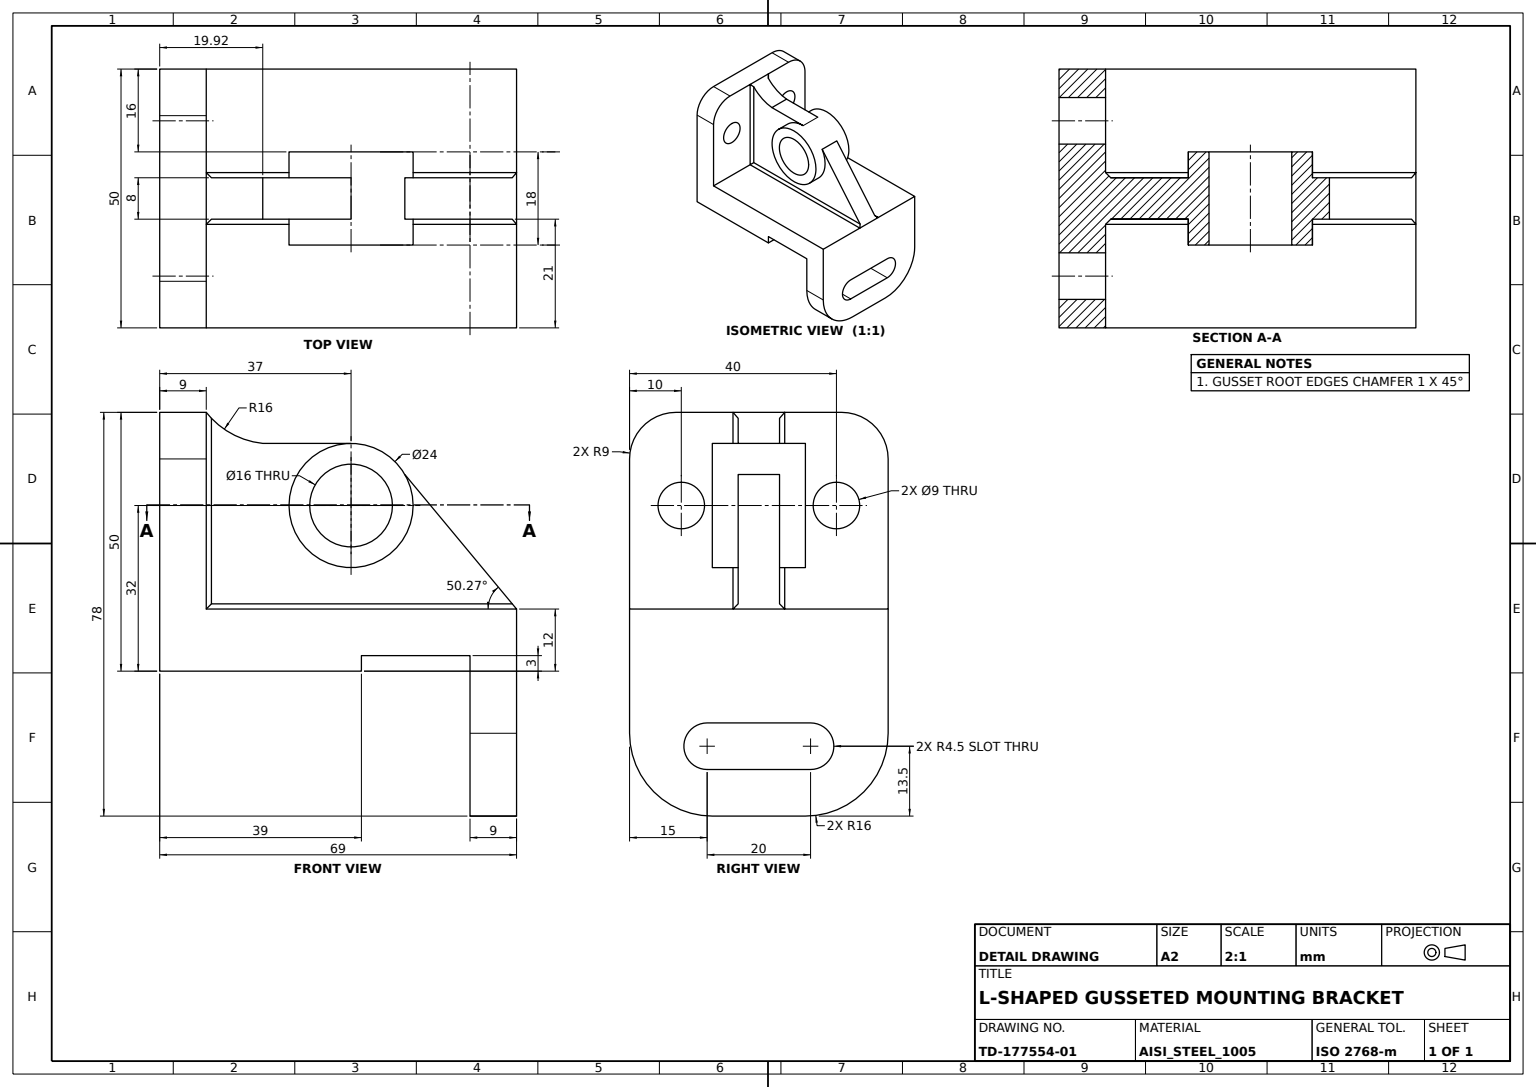
ISO-10303-21;
HEADER;
FILE_DESCRIPTION((''),'2;1');
FILE_NAME('','',(''),(''),'','','');
FILE_SCHEMA(('AUTOMOTIVE_DESIGN'));
ENDSEC;
DATA;
#1=APPLICATION_CONTEXT('');
#2=PRODUCT_CONTEXT('',#1,'mechanical');
#3=PRODUCT('','','',(#2));
#4=PRODUCT_DEFINITION_FORMATION('','',#3);
#5=PRODUCT_DEFINITION_CONTEXT('',#1,'design');
#6=PRODUCT_DEFINITION('','',#4,#5);
#7=PRODUCT_DEFINITION_SHAPE('','',#6);
#8=(LENGTH_UNIT()NAMED_UNIT(*)SI_UNIT(.MILLI.,.METRE.));
#9=(NAMED_UNIT(*)PLANE_ANGLE_UNIT()SI_UNIT($,.RADIAN.));
#10=(NAMED_UNIT(*)SI_UNIT($,.STERADIAN.)SOLID_ANGLE_UNIT());
#11=UNCERTAINTY_MEASURE_WITH_UNIT(LENGTH_MEASURE(0.005),#8,'distance_accuracy_value','');
#12=(GEOMETRIC_REPRESENTATION_CONTEXT(3)GLOBAL_UNCERTAINTY_ASSIGNED_CONTEXT((#11))GLOBAL_UNIT_ASSIGNED_CONTEXT((#8,#9,#10))REPRESENTATION_CONTEXT('',''));
#13=CARTESIAN_POINT('',(9.,-5.,50.));
#14=VERTEX_POINT('',#13);
#15=CARTESIAN_POINT('',(10.,-4.,48.8508));
#16=VERTEX_POINT('',#15);
#17=CARTESIAN_POINT('',(21.556384,7.556384,59.916512));
#18=DIRECTION('',(0.707106781,-0.707106781,0.));
#19=DIRECTION('',(-0.707106781,-0.707106781,0.));
#20=AXIS2_PLACEMENT_3D('',#17,#18,#19);
#21=ELLIPSE('',#20,22.627417,16.);
#22=EDGE_CURVE('',#14,#16,#21,.T.);
#23=ORIENTED_EDGE('',*,*,#22,.F.);
#24=CARTESIAN_POINT('',(9.,-5.,12.));
#25=VERTEX_POINT('',#24);
#26=DIRECTION('',(0.,0.,1.));
#27=VECTOR('',#26,1000.);
#28=LINE('',#13,#27);
#29=EDGE_CURVE('',#25,#14,#28,.T.);
#30=ORIENTED_EDGE('',*,*,#29,.F.);
#31=CARTESIAN_POINT('',(10.,-4.,13.));
#32=VERTEX_POINT('',#31);
#33=CARTESIAN_POINT('',(19.,5.,22.));
#34=DIRECTION('',(0.577350269,0.577350269,0.577350269));
#35=VECTOR('',#34,1000.);
#36=LINE('',#33,#35);
#37=EDGE_CURVE('',#32,#25,#36,.F.);
#38=ORIENTED_EDGE('',*,*,#37,.F.);
#39=CARTESIAN_POINT('',(10.,-4.,12.));
#40=DIRECTION('',(0.,0.,-1.));
#41=VECTOR('',#40,1000.);
#42=LINE('',#39,#41);
#43=EDGE_CURVE('',#16,#32,#42,.T.);
#44=ORIENTED_EDGE('',*,*,#43,.F.);
#45=EDGE_LOOP('',(#23,#30,#38,#44));
#46=FACE_BOUND('',#45,.T.);
#47=CARTESIAN_POINT('',(10.,-4.,32.));
#48=AXIS2_PLACEMENT_3D('',#47,#18,#26);
#49=PLANE('',#48);
#50=ADVANCED_FACE('',(#46),#49,.T.);
#51=CARTESIAN_POINT('',(69.,-9.,-28.));
#52=VERTEX_POINT('',#51);
#53=CARTESIAN_POINT('',(60.,-9.,-28.));
#54=VERTEX_POINT('',#53);
#55=DIRECTION('',(-1.,0.,0.));
#56=VECTOR('',#55,1000.);
#57=LINE('',#51,#56);
#58=EDGE_CURVE('',#52,#54,#57,.T.);
#59=ORIENTED_EDGE('',*,*,#58,.T.);
#60=CARTESIAN_POINT('',(60.,9.,-28.));
#61=VERTEX_POINT('',#60);
#62=DIRECTION('',(0.,1.,0.));
#63=VECTOR('',#62,1000.);
#64=LINE('',#53,#63);
#65=EDGE_CURVE('',#54,#61,#64,.T.);
#66=ORIENTED_EDGE('',*,*,#65,.T.);
#67=CARTESIAN_POINT('',(69.,9.,-28.));
#68=VERTEX_POINT('',#67);
#69=LINE('',#67,#56);
#70=EDGE_CURVE('',#68,#61,#69,.T.);
#71=ORIENTED_EDGE('',*,*,#70,.F.);
#72=LINE('',#51,#63);
#73=EDGE_CURVE('',#52,#68,#72,.T.);
#74=ORIENTED_EDGE('',*,*,#73,.F.);
#75=EDGE_LOOP('',(#59,#66,#71,#74));
#76=FACE_BOUND('',#75,.T.);
#77=DIRECTION('',(1.,0.,0.));
#78=AXIS2_PLACEMENT_3D('',#51,#26,#77);
#79=PLANE('',#78);
#80=ADVANCED_FACE('',(#76),#79,.F.);
#81=CARTESIAN_POINT('',(9.,5.,50.));
#82=VERTEX_POINT('',#81);
#83=CARTESIAN_POINT('',(9.,5.,12.));
#84=VERTEX_POINT('',#83);
#85=LINE('',#83,#41);
#86=EDGE_CURVE('',#82,#84,#85,.T.);
#87=ORIENTED_EDGE('',*,*,#86,.F.);
#88=CARTESIAN_POINT('',(10.,4.,48.8508));
#89=VERTEX_POINT('',#88);
#90=CARTESIAN_POINT('',(21.556384,-7.556384,59.916512));
#91=AXIS2_PLACEMENT_3D('',#90,#19,#18);
#92=ELLIPSE('',#91,22.627417,16.);
#93=EDGE_CURVE('',#89,#82,#92,.F.);
#94=ORIENTED_EDGE('',*,*,#93,.F.);
#95=CARTESIAN_POINT('',(10.,4.,13.));
#96=VERTEX_POINT('',#95);
#97=CARTESIAN_POINT('',(10.,4.,32.));
#98=LINE('',#97,#27);
#99=EDGE_CURVE('',#96,#89,#98,.T.);
#100=ORIENTED_EDGE('',*,*,#99,.F.);
#101=CARTESIAN_POINT('',(26.,-12.,29.));
#102=DIRECTION('',(-0.577350269,0.577350269,-0.577350269));
#103=VECTOR('',#102,1000.);
#104=LINE('',#101,#103);
#105=EDGE_CURVE('',#84,#96,#104,.F.);
#106=ORIENTED_EDGE('',*,*,#105,.F.);
#107=EDGE_LOOP('',(#87,#94,#100,#106));
#108=FACE_BOUND('',#107,.T.);
#109=AXIS2_PLACEMENT_3D('',#83,#19,#40);
#110=PLANE('',#109);
#111=ADVANCED_FACE('',(#108),#110,.F.);
#112=CARTESIAN_POINT('',(69.,10.,-19.));
#113=VERTEX_POINT('',#112);
#114=CARTESIAN_POINT('',(60.,10.,-19.));
#115=VERTEX_POINT('',#114);
#116=LINE('',#112,#56);
#117=EDGE_CURVE('',#113,#115,#116,.T.);
#118=ORIENTED_EDGE('',*,*,#117,.T.);
#119=CARTESIAN_POINT('',(60.,-10.,-19.));
#120=VERTEX_POINT('',#119);
#121=LINE('',#119,#63);
#122=EDGE_CURVE('',#120,#115,#121,.T.);
#123=ORIENTED_EDGE('',*,*,#122,.F.);
#124=CARTESIAN_POINT('',(69.,-10.,-19.));
#125=VERTEX_POINT('',#124);
#126=LINE('',#124,#56);
#127=EDGE_CURVE('',#125,#120,#126,.T.);
#128=ORIENTED_EDGE('',*,*,#127,.F.);
#129=LINE('',#124,#63);
#130=EDGE_CURVE('',#125,#113,#129,.T.);
#131=ORIENTED_EDGE('',*,*,#130,.T.);
#132=EDGE_LOOP('',(#118,#123,#128,#131));
#133=FACE_BOUND('',#132,.T.);
#134=AXIS2_PLACEMENT_3D('',#124,#26,#77);
#135=PLANE('',#134);
#136=ADVANCED_FACE('',(#133),#135,.T.);
#137=CARTESIAN_POINT('',(47.397035,-4.,37.991799));
#138=VERTEX_POINT('',#137);
#139=CARTESIAN_POINT('',(37.,-4.,44.));
#140=VERTEX_POINT('',#139);
#141=CARTESIAN_POINT('',(37.,-4.,32.));
#142=AXIS2_PLACEMENT_3D('',#141,#62,#77);
#143=CIRCLE('',#142,12.);
#144=EDGE_CURVE('',#138,#140,#143,.T.);
#145=ORIENTED_EDGE('',*,*,#144,.T.);
#146=CARTESIAN_POINT('',(19.924011,-4.,44.));
#147=VERTEX_POINT('',#146);
#148=LINE('',#139,#56);
#149=EDGE_CURVE('',#140,#147,#148,.T.);
#150=ORIENTED_EDGE('',*,*,#149,.T.);
#151=CARTESIAN_POINT('',(21.556384,-4.,59.916512));
#152=AXIS2_PLACEMENT_3D('',#151,#62,#77);
#153=CIRCLE('',#152,16.);
#154=EDGE_CURVE('',#147,#16,#153,.T.);
#155=ORIENTED_EDGE('',*,*,#154,.T.);
#156=ORIENTED_EDGE('',*,*,#43,.T.);
#157=CARTESIAN_POINT('',(68.168855,-4.,13.));
#158=VERTEX_POINT('',#157);
#159=CARTESIAN_POINT('',(69.,-4.,13.));
#160=VECTOR('',#77,1000.);
#161=LINE('',#159,#160);
#162=EDGE_CURVE('',#32,#158,#161,.T.);
#163=ORIENTED_EDGE('',*,*,#162,.T.);
#164=CARTESIAN_POINT('',(69.,-4.,12.));
#165=DIRECTION('',(-0.639190848,0.,0.769048152));
#166=VECTOR('',#165,1000.);
#167=LINE('',#164,#166);
#168=EDGE_CURVE('',#158,#138,#167,.T.);
#169=ORIENTED_EDGE('',*,*,#168,.T.);
#170=EDGE_LOOP('',(#145,#150,#155,#156,#163,#169));
#171=FACE_BOUND('',#170,.T.);
#172=AXIS2_PLACEMENT_3D('',#141,#62,#26);
#173=PLANE('',#172);
#174=ADVANCED_FACE('',(#171),#173,.F.);
#175=CARTESIAN_POINT('',(69.,5.,12.));
#176=VERTEX_POINT('',#175);
#177=CARTESIAN_POINT('',(69.,-5.,12.));
#178=VERTEX_POINT('',#177);
#179=CARTESIAN_POINT('',(69.,4.,12.));
#180=DIRECTION('',(0.,-1.,0.));
#181=VECTOR('',#180,1000.);
#182=LINE('',#179,#181);
#183=EDGE_CURVE('',#176,#178,#182,.T.);
#184=ORIENTED_EDGE('',*,*,#183,.T.);
#185=CARTESIAN_POINT('',(69.,-25.,12.));
#186=VERTEX_POINT('',#185);
#187=CARTESIAN_POINT('',(69.,25.,12.));
#188=LINE('',#187,#181);
#189=EDGE_CURVE('',#178,#186,#188,.T.);
#190=ORIENTED_EDGE('',*,*,#189,.T.);
#191=CARTESIAN_POINT('',(69.,-25.,-12.));
#192=VERTEX_POINT('',#191);
#193=LINE('',#185,#41);
#194=EDGE_CURVE('',#186,#192,#193,.T.);
#195=ORIENTED_EDGE('',*,*,#194,.T.);
#196=CARTESIAN_POINT('',(69.,-9.,-12.));
#197=AXIS2_PLACEMENT_3D('',#196,#77,#62);
#198=CIRCLE('',#197,16.);
#199=EDGE_CURVE('',#192,#52,#198,.T.);
#200=ORIENTED_EDGE('',*,*,#199,.T.);
#201=ORIENTED_EDGE('',*,*,#73,.T.);
#202=CARTESIAN_POINT('',(69.,25.,-12.));
#203=VERTEX_POINT('',#202);
#204=CARTESIAN_POINT('',(69.,9.,-12.));
#205=AXIS2_PLACEMENT_3D('',#204,#77,#62);
#206=CIRCLE('',#205,16.);
#207=EDGE_CURVE('',#68,#203,#206,.T.);
#208=ORIENTED_EDGE('',*,*,#207,.T.);
#209=VERTEX_POINT('',#187);
#210=LINE('',#202,#27);
#211=EDGE_CURVE('',#203,#209,#210,.T.);
#212=ORIENTED_EDGE('',*,*,#211,.T.);
#213=EDGE_CURVE('',#209,#176,#188,.T.);
#214=ORIENTED_EDGE('',*,*,#213,.T.);
#215=EDGE_LOOP('',(#184,#190,#195,#200,#201,#208,#212,#214));
#216=FACE_BOUND('',#215,.T.);
#217=CARTESIAN_POINT('',(69.,10.,-10.));
#218=VERTEX_POINT('',#217);
#219=CARTESIAN_POINT('',(69.,10.,-14.5));
#220=AXIS2_PLACEMENT_3D('',#219,#77,#62);
#221=CIRCLE('',#220,4.5);
#222=EDGE_CURVE('',#113,#218,#221,.T.);
#223=ORIENTED_EDGE('',*,*,#222,.F.);
#224=ORIENTED_EDGE('',*,*,#130,.F.);
#225=CARTESIAN_POINT('',(69.,-10.,-10.));
#226=VERTEX_POINT('',#225);
#227=CARTESIAN_POINT('',(69.,-10.,-14.5));
#228=AXIS2_PLACEMENT_3D('',#227,#77,#62);
#229=CIRCLE('',#228,4.5);
#230=EDGE_CURVE('',#226,#125,#229,.T.);
#231=ORIENTED_EDGE('',*,*,#230,.F.);
#232=LINE('',#217,#181);
#233=EDGE_CURVE('',#218,#226,#232,.T.);
#234=ORIENTED_EDGE('',*,*,#233,.F.);
#235=EDGE_LOOP('',(#223,#224,#231,#234));
#236=FACE_BOUND('',#235,.T.);
#237=AXIS2_PLACEMENT_3D('',#196,#77,#40);
#238=PLANE('',#237);
#239=ADVANCED_FACE('',(#216,#236),#238,.T.);
#240=CARTESIAN_POINT('',(60.,-25.,-12.));
#241=VERTEX_POINT('',#240);
#242=CARTESIAN_POINT('',(60.,-9.,-12.));
#243=AXIS2_PLACEMENT_3D('',#242,#77,#62);
#244=CIRCLE('',#243,16.);
#245=EDGE_CURVE('',#241,#54,#244,.T.);
#246=ORIENTED_EDGE('',*,*,#245,.T.);
#247=ORIENTED_EDGE('',*,*,#58,.F.);
#248=ORIENTED_EDGE('',*,*,#199,.F.);
#249=LINE('',#191,#56);
#250=EDGE_CURVE('',#192,#241,#249,.T.);
#251=ORIENTED_EDGE('',*,*,#250,.T.);
#252=EDGE_LOOP('',(#246,#247,#248,#251));
#253=FACE_BOUND('',#252,.T.);
#254=AXIS2_PLACEMENT_3D('',#196,#55,#26);
#255=CYLINDRICAL_SURFACE('',#254,16.);
#256=ADVANCED_FACE('',(#253),#255,.T.);
#257=CARTESIAN_POINT('',(9.,15.,36.5));
#258=VERTEX_POINT('',#257);
#259=CARTESIAN_POINT('',(9.,15.,32.));
#260=AXIS2_PLACEMENT_3D('',#259,#55,#26);
#261=CIRCLE('',#260,4.5);
#262=EDGE_CURVE('',#258,#258,#261,.F.);
#263=ORIENTED_EDGE('',*,*,#262,.T.);
#264=EDGE_LOOP('',(#263));
#265=FACE_BOUND('',#264,.T.);
#266=CARTESIAN_POINT('',(0.,15.,27.5));
#267=VERTEX_POINT('',#266);
#268=CARTESIAN_POINT('',(0.,15.,32.));
#269=AXIS2_PLACEMENT_3D('',#268,#77,#40);
#270=CIRCLE('',#269,4.5);
#271=EDGE_CURVE('',#267,#267,#270,.F.);
#272=ORIENTED_EDGE('',*,*,#271,.T.);
#273=EDGE_LOOP('',(#272));
#274=FACE_BOUND('',#273,.T.);
#275=CARTESIAN_POINT('',(-6.,15.,32.));
#276=AXIS2_PLACEMENT_3D('',#275,#77,#40);
#277=CYLINDRICAL_SURFACE('',#276,4.5);
#278=ADVANCED_FACE('',(#265,#274),#277,.F.);
#279=CARTESIAN_POINT('',(49.,9.,32.));
#280=VERTEX_POINT('',#279);
#281=CARTESIAN_POINT('',(37.,9.,32.));
#282=AXIS2_PLACEMENT_3D('',#281,#180,#77);
#283=CIRCLE('',#282,12.);
#284=EDGE_CURVE('',#280,#280,#283,.T.);
#285=ORIENTED_EDGE('',*,*,#284,.F.);
#286=EDGE_LOOP('',(#285));
#287=FACE_BOUND('',#286,.T.);
#288=CARTESIAN_POINT('',(45.,9.,32.));
#289=VERTEX_POINT('',#288);
#290=CIRCLE('',#282,8.);
#291=EDGE_CURVE('',#289,#289,#290,.T.);
#292=ORIENTED_EDGE('',*,*,#291,.T.);
#293=EDGE_LOOP('',(#292));
#294=FACE_BOUND('',#293,.T.);
#295=AXIS2_PLACEMENT_3D('',#281,#180,#40);
#296=PLANE('',#295);
#297=ADVANCED_FACE('',(#287,#294),#296,.F.);
#298=CARTESIAN_POINT('',(0.,-15.,27.5));
#299=VERTEX_POINT('',#298);
#300=CARTESIAN_POINT('',(0.,-15.,32.));
#301=AXIS2_PLACEMENT_3D('',#300,#77,#40);
#302=CIRCLE('',#301,4.5);
#303=EDGE_CURVE('',#299,#299,#302,.F.);
#304=ORIENTED_EDGE('',*,*,#303,.T.);
#305=EDGE_LOOP('',(#304));
#306=FACE_BOUND('',#305,.T.);
#307=CARTESIAN_POINT('',(9.,-15.,36.5));
#308=VERTEX_POINT('',#307);
#309=CARTESIAN_POINT('',(9.,-15.,32.));
#310=AXIS2_PLACEMENT_3D('',#309,#55,#26);
#311=CIRCLE('',#310,4.5);
#312=EDGE_CURVE('',#308,#308,#311,.F.);
#313=ORIENTED_EDGE('',*,*,#312,.T.);
#314=EDGE_LOOP('',(#313));
#315=FACE_BOUND('',#314,.T.);
#316=CARTESIAN_POINT('',(-6.,-15.,32.));
#317=AXIS2_PLACEMENT_3D('',#316,#77,#40);
#318=CYLINDRICAL_SURFACE('',#317,4.5);
#319=ADVANCED_FACE('',(#306,#315),#318,.F.);
#320=ORIENTED_EDGE('',*,*,#70,.T.);
#321=CARTESIAN_POINT('',(60.,25.,-12.));
#322=VERTEX_POINT('',#321);
#323=CARTESIAN_POINT('',(60.,9.,-12.));
#324=AXIS2_PLACEMENT_3D('',#323,#77,#62);
#325=CIRCLE('',#324,16.);
#326=EDGE_CURVE('',#61,#322,#325,.T.);
#327=ORIENTED_EDGE('',*,*,#326,.T.);
#328=LINE('',#202,#56);
#329=EDGE_CURVE('',#203,#322,#328,.T.);
#330=ORIENTED_EDGE('',*,*,#329,.F.);
#331=ORIENTED_EDGE('',*,*,#207,.F.);
#332=EDGE_LOOP('',(#320,#327,#330,#331));
#333=FACE_BOUND('',#332,.T.);
#334=AXIS2_PLACEMENT_3D('',#204,#55,#26);
#335=CYLINDRICAL_SURFACE('',#334,16.);
#336=ADVANCED_FACE('',(#333),#335,.T.);
#337=CARTESIAN_POINT('',(0.,-25.,41.));
#338=VERTEX_POINT('',#337);
#339=CARTESIAN_POINT('',(0.,-16.,50.));
#340=VERTEX_POINT('',#339);
#341=CARTESIAN_POINT('',(0.,-16.,41.));
#342=AXIS2_PLACEMENT_3D('',#341,#77,#40);
#343=CIRCLE('',#342,9.);
#344=EDGE_CURVE('',#338,#340,#343,.F.);
#345=ORIENTED_EDGE('',*,*,#344,.T.);
#346=CARTESIAN_POINT('',(0.,16.,50.));
#347=VERTEX_POINT('',#346);
#348=CARTESIAN_POINT('',(0.,-25.,50.));
#349=LINE('',#348,#63);
#350=EDGE_CURVE('',#340,#347,#349,.T.);
#351=ORIENTED_EDGE('',*,*,#350,.T.);
#352=CARTESIAN_POINT('',(0.,25.,41.));
#353=VERTEX_POINT('',#352);
#354=CARTESIAN_POINT('',(0.,16.,41.));
#355=AXIS2_PLACEMENT_3D('',#354,#77,#40);
#356=CIRCLE('',#355,9.);
#357=EDGE_CURVE('',#347,#353,#356,.F.);
#358=ORIENTED_EDGE('',*,*,#357,.T.);
#359=CARTESIAN_POINT('',(0.,25.,0.));
#360=VERTEX_POINT('',#359);
#361=CARTESIAN_POINT('',(0.,25.,50.));
#362=LINE('',#361,#41);
#363=EDGE_CURVE('',#353,#360,#362,.T.);
#364=ORIENTED_EDGE('',*,*,#363,.T.);
#365=CARTESIAN_POINT('',(0.,-25.,0.));
#366=VERTEX_POINT('',#365);
#367=LINE('',#365,#63);
#368=EDGE_CURVE('',#366,#360,#367,.T.);
#369=ORIENTED_EDGE('',*,*,#368,.F.);
#370=LINE('',#348,#41);
#371=EDGE_CURVE('',#338,#366,#370,.T.);
#372=ORIENTED_EDGE('',*,*,#371,.F.);
#373=EDGE_LOOP('',(#345,#351,#358,#364,#369,#372));
#374=FACE_BOUND('',#373,.T.);
#375=ORIENTED_EDGE('',*,*,#303,.F.);
#376=EDGE_LOOP('',(#375));
#377=FACE_BOUND('',#376,.T.);
#378=ORIENTED_EDGE('',*,*,#271,.F.);
#379=EDGE_LOOP('',(#378));
#380=FACE_BOUND('',#379,.T.);
#381=AXIS2_PLACEMENT_3D('',#348,#77,#40);
#382=PLANE('',#381);
#383=ADVANCED_FACE('',(#374,#377,#380),#382,.F.);
#384=CARTESIAN_POINT('',(60.,10.,-10.));
#385=VERTEX_POINT('',#384);
#386=CARTESIAN_POINT('',(60.,-10.,-10.));
#387=VERTEX_POINT('',#386);
#388=LINE('',#384,#181);
#389=EDGE_CURVE('',#385,#387,#388,.T.);
#390=ORIENTED_EDGE('',*,*,#389,.F.);
#391=LINE('',#217,#56);
#392=EDGE_CURVE('',#218,#385,#391,.T.);
#393=ORIENTED_EDGE('',*,*,#392,.F.);
#394=ORIENTED_EDGE('',*,*,#233,.T.);
#395=LINE('',#225,#56);
#396=EDGE_CURVE('',#226,#387,#395,.T.);
#397=ORIENTED_EDGE('',*,*,#396,.T.);
#398=EDGE_LOOP('',(#390,#393,#394,#397));
#399=FACE_BOUND('',#398,.T.);
#400=AXIS2_PLACEMENT_3D('',#217,#40,#55);
#401=PLANE('',#400);
#402=ADVANCED_FACE('',(#399),#401,.T.);
#403=ORIENTED_EDGE('',*,*,#329,.T.);
#404=CARTESIAN_POINT('',(60.,25.,3.));
#405=VERTEX_POINT('',#404);
#406=LINE('',#321,#27);
#407=EDGE_CURVE('',#322,#405,#406,.T.);
#408=ORIENTED_EDGE('',*,*,#407,.T.);
#409=CARTESIAN_POINT('',(39.,25.,3.));
#410=VERTEX_POINT('',#409);
#411=LINE('',#409,#160);
#412=EDGE_CURVE('',#410,#405,#411,.T.);
#413=ORIENTED_EDGE('',*,*,#412,.F.);
#414=CARTESIAN_POINT('',(39.,25.,0.));
#415=VERTEX_POINT('',#414);
#416=LINE('',#414,#27);
#417=EDGE_CURVE('',#415,#410,#416,.T.);
#418=ORIENTED_EDGE('',*,*,#417,.F.);
#419=LINE('',#359,#160);
#420=EDGE_CURVE('',#360,#415,#419,.T.);
#421=ORIENTED_EDGE('',*,*,#420,.F.);
#422=ORIENTED_EDGE('',*,*,#363,.F.);
#423=CARTESIAN_POINT('',(9.,25.,41.));
#424=VERTEX_POINT('',#423);
#425=LINE('',#352,#56);
#426=EDGE_CURVE('',#353,#424,#425,.F.);
#427=ORIENTED_EDGE('',*,*,#426,.T.);
#428=CARTESIAN_POINT('',(9.,25.,12.));
#429=VERTEX_POINT('',#428);
#430=LINE('',#428,#27);
#431=EDGE_CURVE('',#429,#424,#430,.T.);
#432=ORIENTED_EDGE('',*,*,#431,.F.);
#433=CARTESIAN_POINT('',(60.,25.,12.));
#434=LINE('',#433,#56);
#435=EDGE_CURVE('',#209,#429,#434,.T.);
#436=ORIENTED_EDGE('',*,*,#435,.F.);
#437=ORIENTED_EDGE('',*,*,#211,.F.);
#438=EDGE_LOOP('',(#403,#408,#413,#418,#421,#422,#427,#432,#436,#437));
#439=FACE_BOUND('',#438,.T.);
#440=AXIS2_PLACEMENT_3D('',#359,#180,#40);
#441=PLANE('',#440);
#442=ADVANCED_FACE('',(#439),#441,.F.);
#443=CARTESIAN_POINT('',(68.168855,4.,13.));
#444=VERTEX_POINT('',#443);
#445=CARTESIAN_POINT('',(47.397035,4.,37.991799));
#446=VERTEX_POINT('',#445);
#447=LINE('',#179,#166);
#448=EDGE_CURVE('',#444,#446,#447,.T.);
#449=ORIENTED_EDGE('',*,*,#448,.T.);
#450=LINE('',#445,#181);
#451=EDGE_CURVE('',#446,#138,#450,.T.);
#452=ORIENTED_EDGE('',*,*,#451,.T.);
#453=ORIENTED_EDGE('',*,*,#168,.F.);
#454=CARTESIAN_POINT('',(60.166956,5.627555,22.627555));
#455=DIRECTION('',(-0.506682713,0.609619811,0.609619811));
#456=VECTOR('',#455,1000.);
#457=LINE('',#454,#456);
#458=EDGE_CURVE('',#158,#178,#457,.F.);
#459=ORIENTED_EDGE('',*,*,#458,.T.);
#460=ORIENTED_EDGE('',*,*,#183,.F.);
#461=CARTESIAN_POINT('',(66.689454,2.220046,14.779954));
#462=DIRECTION('',(-0.506682713,-0.609619811,0.609619811));
#463=VECTOR('',#462,1000.);
#464=LINE('',#461,#463);
#465=EDGE_CURVE('',#176,#444,#464,.T.);
#466=ORIENTED_EDGE('',*,*,#465,.T.);
#467=EDGE_LOOP('',(#449,#452,#453,#459,#460,#466));
#468=FACE_BOUND('',#467,.T.);
#469=DIRECTION('',(0.769048152,0.,0.639190848));
#470=DIRECTION('',(0.639190848,0.,-0.769048152));
#471=AXIS2_PLACEMENT_3D('',#179,#469,#470);
#472=PLANE('',#471);
#473=ADVANCED_FACE('',(#468),#472,.T.);
#474=CARTESIAN_POINT('',(39.,-25.,0.));
#475=VERTEX_POINT('',#474);
#476=CARTESIAN_POINT('',(39.,-25.,3.));
#477=VERTEX_POINT('',#476);
#478=LINE('',#474,#27);
#479=EDGE_CURVE('',#475,#477,#478,.T.);
#480=ORIENTED_EDGE('',*,*,#479,.F.);
#481=LINE('',#474,#63);
#482=EDGE_CURVE('',#475,#415,#481,.T.);
#483=ORIENTED_EDGE('',*,*,#482,.T.);
#484=ORIENTED_EDGE('',*,*,#417,.T.);
#485=LINE('',#476,#63);
#486=EDGE_CURVE('',#477,#410,#485,.T.);
#487=ORIENTED_EDGE('',*,*,#486,.F.);
#488=EDGE_LOOP('',(#480,#483,#484,#487));
#489=FACE_BOUND('',#488,.T.);
#490=AXIS2_PLACEMENT_3D('',#474,#55,#26);
#491=PLANE('',#490);
#492=ADVANCED_FACE('',(#489),#491,.F.);
#493=CARTESIAN_POINT('',(37.,4.,44.));
#494=VERTEX_POINT('',#493);
#495=CARTESIAN_POINT('',(37.,4.,32.));
#496=AXIS2_PLACEMENT_3D('',#495,#62,#77);
#497=CIRCLE('',#496,12.);
#498=EDGE_CURVE('',#446,#494,#497,.T.);
#499=ORIENTED_EDGE('',*,*,#498,.T.);
#500=LINE('',#493,#181);
#501=EDGE_CURVE('',#494,#140,#500,.T.);
#502=ORIENTED_EDGE('',*,*,#501,.T.);
#503=ORIENTED_EDGE('',*,*,#144,.F.);
#504=ORIENTED_EDGE('',*,*,#451,.F.);
#505=EDGE_LOOP('',(#499,#502,#503,#504));
#506=FACE_BOUND('',#505,.T.);
#507=ORIENTED_EDGE('',*,*,#284,.T.);
#508=EDGE_LOOP('',(#507));
#509=FACE_BOUND('',#508,.T.);
#510=CARTESIAN_POINT('',(49.,-9.,32.));
#511=VERTEX_POINT('',#510);
#512=CARTESIAN_POINT('',(37.,-9.,32.));
#513=AXIS2_PLACEMENT_3D('',#512,#180,#77);
#514=CIRCLE('',#513,12.);
#515=EDGE_CURVE('',#511,#511,#514,.T.);
#516=ORIENTED_EDGE('',*,*,#515,.F.);
#517=EDGE_LOOP('',(#516));
#518=FACE_BOUND('',#517,.T.);
#519=AXIS2_PLACEMENT_3D('',#512,#62,#26);
#520=CYLINDRICAL_SURFACE('',#519,12.);
#521=ADVANCED_FACE('',(#506,#509,#518),#520,.T.);
#522=CARTESIAN_POINT('',(45.,-9.,32.));
#523=VERTEX_POINT('',#522);
#524=CIRCLE('',#513,8.);
#525=EDGE_CURVE('',#523,#523,#524,.T.);
#526=ORIENTED_EDGE('',*,*,#525,.T.);
#527=EDGE_LOOP('',(#526));
#528=FACE_BOUND('',#527,.T.);
#529=ORIENTED_EDGE('',*,*,#291,.F.);
#530=EDGE_LOOP('',(#529));
#531=FACE_BOUND('',#530,.T.);
#532=CYLINDRICAL_SURFACE('',#519,8.);
#533=ADVANCED_FACE('',(#528,#531),#532,.F.);
#534=CARTESIAN_POINT('',(60.,10.,-14.5));
#535=AXIS2_PLACEMENT_3D('',#534,#77,#62);
#536=CIRCLE('',#535,4.5);
#537=EDGE_CURVE('',#115,#385,#536,.T.);
#538=ORIENTED_EDGE('',*,*,#537,.T.);
#539=ORIENTED_EDGE('',*,*,#389,.T.);
#540=CARTESIAN_POINT('',(60.,-10.,-14.5));
#541=AXIS2_PLACEMENT_3D('',#540,#77,#62);
#542=CIRCLE('',#541,4.5);
#543=EDGE_CURVE('',#387,#120,#542,.T.);
#544=ORIENTED_EDGE('',*,*,#543,.T.);
#545=ORIENTED_EDGE('',*,*,#122,.T.);
#546=EDGE_LOOP('',(#538,#539,#544,#545));
#547=FACE_BOUND('',#546,.T.);
#548=ORIENTED_EDGE('',*,*,#407,.F.);
#549=ORIENTED_EDGE('',*,*,#326,.F.);
#550=ORIENTED_EDGE('',*,*,#65,.F.);
#551=ORIENTED_EDGE('',*,*,#245,.F.);
#552=CARTESIAN_POINT('',(60.,-25.,3.));
#553=VERTEX_POINT('',#552);
#554=CARTESIAN_POINT('',(60.,-25.,12.));
#555=LINE('',#554,#41);
#556=EDGE_CURVE('',#553,#241,#555,.T.);
#557=ORIENTED_EDGE('',*,*,#556,.F.);
#558=LINE('',#552,#63);
#559=EDGE_CURVE('',#553,#405,#558,.T.);
#560=ORIENTED_EDGE('',*,*,#559,.T.);
#561=EDGE_LOOP('',(#548,#549,#550,#551,#557,#560));
#562=FACE_BOUND('',#561,.T.);
#563=AXIS2_PLACEMENT_3D('',#242,#77,#40);
#564=PLANE('',#563);
#565=ADVANCED_FACE('',(#547,#562),#564,.F.);
#566=ORIENTED_EDGE('',*,*,#213,.F.);
#567=ORIENTED_EDGE('',*,*,#435,.T.);
#568=CARTESIAN_POINT('',(9.,-25.,12.));
#569=LINE('',#568,#63);
#570=EDGE_CURVE('',#84,#429,#569,.T.);
#571=ORIENTED_EDGE('',*,*,#570,.F.);
#572=CARTESIAN_POINT('',(60.,5.,12.));
#573=LINE('',#572,#160);
#574=EDGE_CURVE('',#84,#176,#573,.T.);
#575=ORIENTED_EDGE('',*,*,#574,.T.);
#576=EDGE_LOOP('',(#566,#567,#571,#575));
#577=FACE_BOUND('',#576,.T.);
#578=AXIS2_PLACEMENT_3D('',#554,#40,#55);
#579=PLANE('',#578);
#580=ADVANCED_FACE('',(#577),#579,.F.);
#581=CARTESIAN_POINT('',(9.,-25.,41.));
#582=VERTEX_POINT('',#581);
#583=LINE('',#337,#56);
#584=EDGE_CURVE('',#582,#338,#583,.T.);
#585=ORIENTED_EDGE('',*,*,#584,.F.);
#586=CARTESIAN_POINT('',(9.,-16.,50.));
#587=VERTEX_POINT('',#586);
#588=CARTESIAN_POINT('',(9.,-16.,41.));
#589=AXIS2_PLACEMENT_3D('',#588,#55,#26);
#590=CIRCLE('',#589,9.);
#591=EDGE_CURVE('',#587,#582,#590,.F.);
#592=ORIENTED_EDGE('',*,*,#591,.F.);
#593=LINE('',#586,#56);
#594=EDGE_CURVE('',#340,#587,#593,.F.);
#595=ORIENTED_EDGE('',*,*,#594,.F.);
#596=ORIENTED_EDGE('',*,*,#344,.F.);
#597=EDGE_LOOP('',(#585,#592,#595,#596));
#598=FACE_BOUND('',#597,.T.);
#599=CYLINDRICAL_SURFACE('',#342,9.);
#600=ADVANCED_FACE('',(#598),#599,.T.);
#601=ORIENTED_EDGE('',*,*,#396,.F.);
#602=ORIENTED_EDGE('',*,*,#230,.T.);
#603=ORIENTED_EDGE('',*,*,#127,.T.);
#604=ORIENTED_EDGE('',*,*,#543,.F.);
#605=EDGE_LOOP('',(#601,#602,#603,#604));
#606=FACE_BOUND('',#605,.T.);
#607=AXIS2_PLACEMENT_3D('',#227,#55,#26);
#608=CYLINDRICAL_SURFACE('',#607,4.5);
#609=ADVANCED_FACE('',(#606),#608,.F.);
#610=ORIENTED_EDGE('',*,*,#262,.F.);
#611=EDGE_LOOP('',(#610));
#612=FACE_BOUND('',#611,.T.);
#613=ORIENTED_EDGE('',*,*,#86,.T.);
#614=ORIENTED_EDGE('',*,*,#570,.T.);
#615=ORIENTED_EDGE('',*,*,#431,.T.);
#616=CARTESIAN_POINT('',(9.,16.,50.));
#617=VERTEX_POINT('',#616);
#618=CARTESIAN_POINT('',(9.,16.,41.));
#619=AXIS2_PLACEMENT_3D('',#618,#55,#26);
#620=CIRCLE('',#619,9.);
#621=EDGE_CURVE('',#424,#617,#620,.F.);
#622=ORIENTED_EDGE('',*,*,#621,.T.);
#623=CARTESIAN_POINT('',(9.,-25.,50.));
#624=LINE('',#623,#63);
#625=EDGE_CURVE('',#82,#617,#624,.T.);
#626=ORIENTED_EDGE('',*,*,#625,.F.);
#627=EDGE_LOOP('',(#613,#614,#615,#622,#626));
#628=FACE_BOUND('',#627,.T.);
#629=AXIS2_PLACEMENT_3D('',#568,#55,#26);
#630=PLANE('',#629);
#631=ADVANCED_FACE('',(#612,#628),#630,.F.);
#632=ORIENTED_EDGE('',*,*,#621,.F.);
#633=ORIENTED_EDGE('',*,*,#426,.F.);
#634=ORIENTED_EDGE('',*,*,#357,.F.);
#635=LINE('',#616,#56);
#636=EDGE_CURVE('',#617,#347,#635,.T.);
#637=ORIENTED_EDGE('',*,*,#636,.F.);
#638=EDGE_LOOP('',(#632,#633,#634,#637));
#639=FACE_BOUND('',#638,.T.);
#640=CYLINDRICAL_SURFACE('',#619,9.);
#641=ADVANCED_FACE('',(#639),#640,.T.);
#642=ORIENTED_EDGE('',*,*,#368,.T.);
#643=ORIENTED_EDGE('',*,*,#420,.T.);
#644=ORIENTED_EDGE('',*,*,#482,.F.);
#645=LINE('',#365,#160);
#646=EDGE_CURVE('',#366,#475,#645,.T.);
#647=ORIENTED_EDGE('',*,*,#646,.F.);
#648=EDGE_LOOP('',(#642,#643,#644,#647));
#649=FACE_BOUND('',#648,.T.);
#650=AXIS2_PLACEMENT_3D('',#365,#26,#77);
#651=PLANE('',#650);
#652=ADVANCED_FACE('',(#649),#651,.F.);
#653=LINE('',#476,#160);
#654=EDGE_CURVE('',#477,#553,#653,.T.);
#655=ORIENTED_EDGE('',*,*,#654,.F.);
#656=ORIENTED_EDGE('',*,*,#486,.T.);
#657=ORIENTED_EDGE('',*,*,#412,.T.);
#658=ORIENTED_EDGE('',*,*,#559,.F.);
#659=EDGE_LOOP('',(#655,#656,#657,#658));
#660=FACE_BOUND('',#659,.T.);
#661=AXIS2_PLACEMENT_3D('',#476,#26,#77);
#662=PLANE('',#661);
#663=ADVANCED_FACE('',(#660),#662,.F.);
#664=ORIENTED_EDGE('',*,*,#222,.T.);
#665=ORIENTED_EDGE('',*,*,#392,.T.);
#666=ORIENTED_EDGE('',*,*,#537,.F.);
#667=ORIENTED_EDGE('',*,*,#117,.F.);
#668=EDGE_LOOP('',(#664,#665,#666,#667));
#669=FACE_BOUND('',#668,.T.);
#670=AXIS2_PLACEMENT_3D('',#219,#55,#26);
#671=CYLINDRICAL_SURFACE('',#670,4.5);
#672=ADVANCED_FACE('',(#669),#671,.F.);
#673=ORIENTED_EDGE('',*,*,#574,.F.);
#674=ORIENTED_EDGE('',*,*,#105,.T.);
#675=CARTESIAN_POINT('',(37.,4.,13.));
#676=LINE('',#675,#56);
#677=EDGE_CURVE('',#444,#96,#676,.T.);
#678=ORIENTED_EDGE('',*,*,#677,.F.);
#679=ORIENTED_EDGE('',*,*,#465,.F.);
#680=EDGE_LOOP('',(#673,#674,#678,#679));
#681=FACE_BOUND('',#680,.T.);
#682=DIRECTION('',(0.,-0.707106781,-0.707106781));
#683=AXIS2_PLACEMENT_3D('',#572,#682,#77);
#684=PLANE('',#683);
#685=ADVANCED_FACE('',(#681),#684,.F.);
#686=ORIENTED_EDGE('',*,*,#350,.F.);
#687=ORIENTED_EDGE('',*,*,#594,.T.);
#688=EDGE_CURVE('',#587,#14,#624,.T.);
#689=ORIENTED_EDGE('',*,*,#688,.T.);
#690=CARTESIAN_POINT('',(9.,4.,50.));
#691=LINE('',#690,#181);
#692=EDGE_CURVE('',#82,#14,#691,.T.);
#693=ORIENTED_EDGE('',*,*,#692,.F.);
#694=ORIENTED_EDGE('',*,*,#625,.T.);
#695=ORIENTED_EDGE('',*,*,#636,.T.);
#696=EDGE_LOOP('',(#686,#687,#689,#693,#694,#695));
#697=FACE_BOUND('',#696,.T.);
#698=AXIS2_PLACEMENT_3D('',#623,#40,#55);
#699=PLANE('',#698);
#700=ADVANCED_FACE('',(#697),#699,.F.);
#701=ORIENTED_EDGE('',*,*,#250,.F.);
#702=ORIENTED_EDGE('',*,*,#194,.F.);
#703=VERTEX_POINT('',#568);
#704=LINE('',#554,#56);
#705=EDGE_CURVE('',#186,#703,#704,.T.);
#706=ORIENTED_EDGE('',*,*,#705,.T.);
#707=LINE('',#568,#27);
#708=EDGE_CURVE('',#703,#582,#707,.T.);
#709=ORIENTED_EDGE('',*,*,#708,.T.);
#710=ORIENTED_EDGE('',*,*,#584,.T.);
#711=ORIENTED_EDGE('',*,*,#371,.T.);
#712=ORIENTED_EDGE('',*,*,#646,.T.);
#713=ORIENTED_EDGE('',*,*,#479,.T.);
#714=ORIENTED_EDGE('',*,*,#654,.T.);
#715=ORIENTED_EDGE('',*,*,#556,.T.);
#716=EDGE_LOOP('',(#701,#702,#706,#709,#710,#711,#712,#713,#714,#715));
#717=FACE_BOUND('',#716,.T.);
#718=AXIS2_PLACEMENT_3D('',#365,#180,#40);
#719=PLANE('',#718);
#720=ADVANCED_FACE('',(#717),#719,.T.);
#721=CARTESIAN_POINT('',(19.924011,4.,44.));
#722=VERTEX_POINT('',#721);
#723=LINE('',#493,#56);
#724=EDGE_CURVE('',#494,#722,#723,.T.);
#725=ORIENTED_EDGE('',*,*,#724,.T.);
#726=LINE('',#721,#181);
#727=EDGE_CURVE('',#722,#147,#726,.T.);
#728=ORIENTED_EDGE('',*,*,#727,.T.);
#729=ORIENTED_EDGE('',*,*,#149,.F.);
#730=ORIENTED_EDGE('',*,*,#501,.F.);
#731=EDGE_LOOP('',(#725,#728,#729,#730));
#732=FACE_BOUND('',#731,.T.);
#733=AXIS2_PLACEMENT_3D('',#493,#26,#77);
#734=PLANE('',#733);
#735=ADVANCED_FACE('',(#732),#734,.T.);
#736=ORIENTED_EDGE('',*,*,#525,.F.);
#737=EDGE_LOOP('',(#736));
#738=FACE_BOUND('',#737,.T.);
#739=ORIENTED_EDGE('',*,*,#515,.T.);
#740=EDGE_LOOP('',(#739));
#741=FACE_BOUND('',#740,.T.);
#742=AXIS2_PLACEMENT_3D('',#512,#180,#40);
#743=PLANE('',#742);
#744=ADVANCED_FACE('',(#738,#741),#743,.T.);
#745=CARTESIAN_POINT('',(21.556384,4.,59.916512));
#746=AXIS2_PLACEMENT_3D('',#745,#62,#77);
#747=CIRCLE('',#746,16.);
#748=EDGE_CURVE('',#722,#89,#747,.T.);
#749=ORIENTED_EDGE('',*,*,#748,.T.);
#750=ORIENTED_EDGE('',*,*,#93,.T.);
#751=ORIENTED_EDGE('',*,*,#692,.T.);
#752=ORIENTED_EDGE('',*,*,#22,.T.);
#753=ORIENTED_EDGE('',*,*,#154,.F.);
#754=ORIENTED_EDGE('',*,*,#727,.F.);
#755=EDGE_LOOP('',(#749,#750,#751,#752,#753,#754));
#756=FACE_BOUND('',#755,.T.);
#757=AXIS2_PLACEMENT_3D('',#745,#180,#40);
#758=CYLINDRICAL_SURFACE('',#757,16.);
#759=ADVANCED_FACE('',(#756),#758,.F.);
#760=LINE('',#24,#56);
#761=EDGE_CURVE('',#178,#25,#760,.T.);
#762=ORIENTED_EDGE('',*,*,#761,.T.);
#763=EDGE_CURVE('',#703,#25,#569,.T.);
#764=ORIENTED_EDGE('',*,*,#763,.F.);
#765=ORIENTED_EDGE('',*,*,#705,.F.);
#766=ORIENTED_EDGE('',*,*,#189,.F.);
#767=EDGE_LOOP('',(#762,#764,#765,#766));
#768=FACE_BOUND('',#767,.T.);
#769=ADVANCED_FACE('',(#768),#579,.F.);
#770=ORIENTED_EDGE('',*,*,#312,.F.);
#771=EDGE_LOOP('',(#770));
#772=FACE_BOUND('',#771,.T.);
#773=ORIENTED_EDGE('',*,*,#29,.T.);
#774=ORIENTED_EDGE('',*,*,#688,.F.);
#775=ORIENTED_EDGE('',*,*,#591,.T.);
#776=ORIENTED_EDGE('',*,*,#708,.F.);
#777=ORIENTED_EDGE('',*,*,#763,.T.);
#778=EDGE_LOOP('',(#773,#774,#775,#776,#777));
#779=FACE_BOUND('',#778,.T.);
#780=ADVANCED_FACE('',(#772,#779),#630,.F.);
#781=ORIENTED_EDGE('',*,*,#748,.F.);
#782=ORIENTED_EDGE('',*,*,#724,.F.);
#783=ORIENTED_EDGE('',*,*,#498,.F.);
#784=ORIENTED_EDGE('',*,*,#448,.F.);
#785=ORIENTED_EDGE('',*,*,#677,.T.);
#786=ORIENTED_EDGE('',*,*,#99,.T.);
#787=EDGE_LOOP('',(#781,#782,#783,#784,#785,#786));
#788=FACE_BOUND('',#787,.T.);
#789=AXIS2_PLACEMENT_3D('',#495,#62,#26);
#790=PLANE('',#789);
#791=ADVANCED_FACE('',(#788),#790,.T.);
#792=ORIENTED_EDGE('',*,*,#37,.T.);
#793=ORIENTED_EDGE('',*,*,#761,.F.);
#794=ORIENTED_EDGE('',*,*,#458,.F.);
#795=ORIENTED_EDGE('',*,*,#162,.F.);
#796=EDGE_LOOP('',(#792,#793,#794,#795));
#797=FACE_BOUND('',#796,.T.);
#798=CARTESIAN_POINT('',(37.,-4.,13.));
#799=DIRECTION('',(0.,-0.707106781,0.707106781));
#800=AXIS2_PLACEMENT_3D('',#798,#799,#55);
#801=PLANE('',#800);
#802=ADVANCED_FACE('',(#797),#801,.T.);
#803=CLOSED_SHELL('',(#50,#80,#111,#136,#174,#239,#256,#278,#297,#319,#336,#383,#402,#442,#473,#492,#521,#533,#565,#580,#600,#609,#631,#641,#652,#663,#672,#685,#700,#720,#735,#744,#759,#769,#780,#791,#802));
#804=MANIFOLD_SOLID_BREP('',#803);
#805=ADVANCED_BREP_SHAPE_REPRESENTATION('',(#804),#12);
#806=SHAPE_DEFINITION_REPRESENTATION(#7,#805);
ENDSEC;
END-ISO-10303-21;
